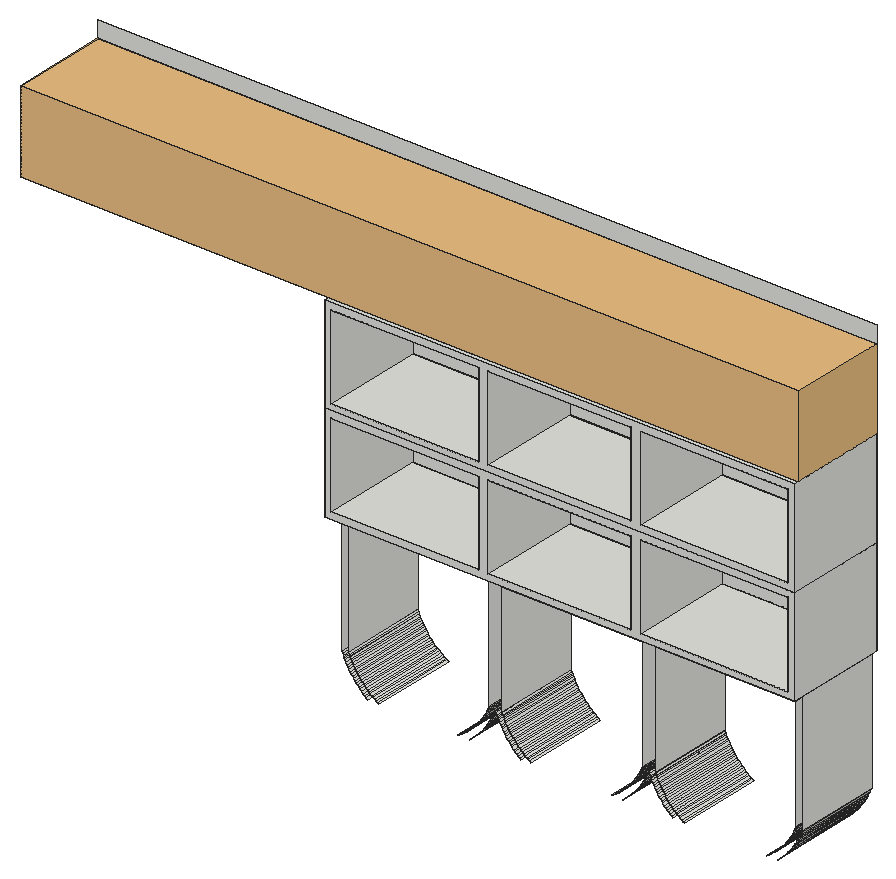
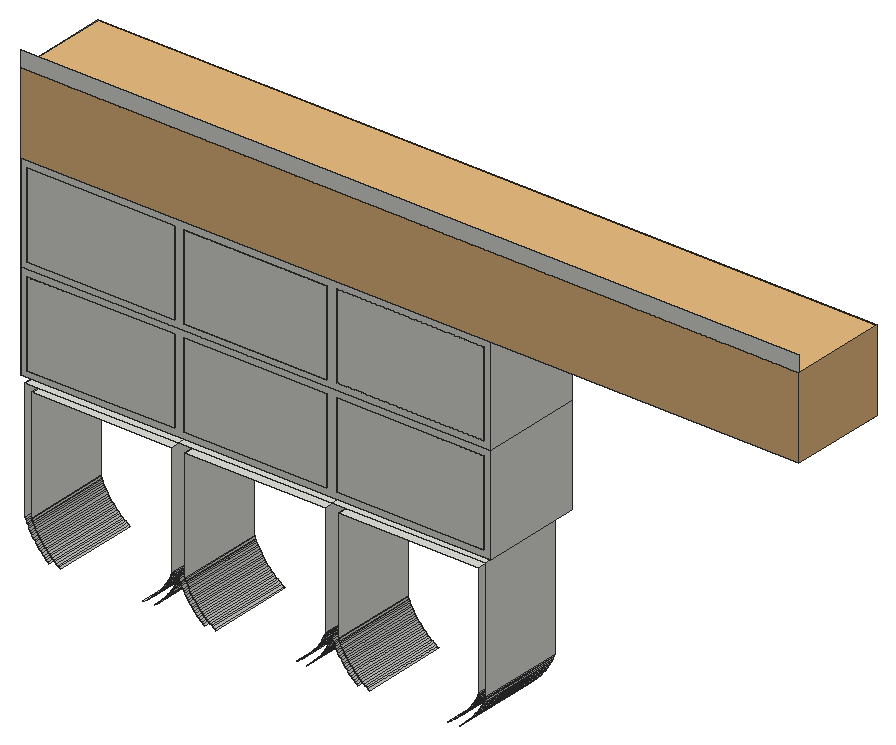
# SketchUp Ruby script. Lengths in inches.
U = 1.inch
M = Sketchup.active_model
def pt(a) = Geom::Point3d.new(a.map { |v| v * U })
def face(e, loops, mat)
  f = e.add_face(loops[0].map { |a| pt(a) })
  loops[1..].each { |l| e.add_face(l.map { |a| pt(a) }).erase! }
  f.material = f.back_material = mat if mat
  f
end
# faces: each face lists its corners as indices into pts; further lists are holes
def faces(e, pts, list, mat = nil) = list.each { |f| face(e, (f[0].is_a?(Array) ? f : [f]).map { |l| l.map { |i| pts[i] } }, mat) }
# xy, xz, yz: faces in a plane at the given z, y or x. An outline is a flat list of corners, or four numbers for a rectangle; further outlines are holes
def ring(l) = l.size == 4 ? [[l[0], l[1]], [l[2], l[1]], [l[2], l[3]], [l[0], l[3]]] : l.each_slice(2).to_a
def flat(e, list, mat, &to3) = list.each { |f| face(e, (f[0].is_a?(Array) ? f : [f]).map { |l| ring(l).map { |u, v| to3.(u, v) } }, mat) }
def xy(e, z, list, mat = nil) = flat(e, list, mat) { |x, y| [x, y, z] }
def xz(e, y, list, mat = nil) = flat(e, list, mat) { |x, z| [x, y, z] }
def yz(e, x, list, mat = nil) = flat(e, list, mat) { |y, z| [x, y, z] }
def lines(e, pts, list) = list.each { |a, b| e.add_line(pt(pts[a]), pt(pts[b])) }
# prism: a flat outline (further loops are holes) pulled along v
def prism(e, loops, v, mat = nil)
  f = face(e, loops, mat); d = Geom::Vector3d.new(v.map { |x| x * U })
  f.pushpull(f.normal.samedirection?(d) ? d.length : -d.length)
end
def box(e, o, s, mat = nil) = prism(e, [[o, [o[0] + s[0], o[1], o[2]], [o[0] + s[0], o[1] + s[1], o[2]], [o[0], o[1] + s[1], o[2]]]], [0, 0, s[2]], mat)
def at(x, y, z, deg = 0) = Geom::Transformation.translation(pt([x, y, z])) * Geom::Transformation.rotation(ORIGIN, Z_AXIS, deg.degrees)
def axes(o, x, y, z) = Geom::Transformation.new([*x, 0, *y, 0, *z, 0, *pt(o).to_a, 1])
def part(name) = M.definitions.add(name)
# library, detail: a bought-in or finely detailed component or shape, given as its bounding box
def library(name, o, s) = part(name).tap { |d| box(d.entities, o, s) }
def detail(e, o, s) = box(e.add_group.entities, o, s)
def put(e, d, t, mat = nil) = e.add_instance(d, t).tap { |i| i.material = mat if mat }
def group(e, t, mat = nil) = e.add_group.tap { |g| g.transformation = t; g.material = mat if mat }.entities
root = M.entities
c1 = library("Group\#5",[0,-12,0],[96,12,10])
xy(root,82.6,[[45.4,19.34,62.73,30],[64.33,19.34,81.67,30],[83.27,19.34,100.6,30]])
xy(root,83.4,[[44.6,19.34,63.53,30],[63.53,19.34,82.47,30],[82.47,19.34,101.4,30]])
xz(root,30,[[44.8,84.8,63,95.2],[64.2,84.8,81.8,95.2],[83,84.8,101.2,95.2],[6,118,102,120]])
yz(root,44.6,[[19.34,68.6,30,83.4]])
yz(root,45.4,[[19.34,68.75,30,82.6]])
yz(root,62.73,[[19.34,68.75,30,82.6]])
yz(root,64.33,[[19.34,68.75,30,82.6]])
yz(root,81.67,[[19.34,68.75,30,82.6]])
yz(root,83.27,[[19.34,68.75,30,82.6]])
yz(root,100.6,[[19.34,68.75,30,82.6]])
yz(root,101.4,[[19.34,68.6,30,83.4]])
p = [[47.59,30,64.45],[47.78,30,64.29],[47.78,19.34,64.29],[47.59,19.34,64.45],[49.21,30,64.28],[49.02,30,64.4],
  [49.02,19.34,64.4],[49.21,19.34,64.28],[59.11,30,64.4],[58.92,30,64.28],[58.92,19.34,64.28],[59.11,19.34,64.4],
  [60.35,30,64.29],[60.54,30,64.45],[60.54,19.34,64.45],[60.35,19.34,64.29],[66.52,30,64.4375],[66.71,30,64.28],
  [66.71,19.34,64.28],[66.52,19.34,64.4375],[78.05,30,64.38],[77.86,30,64.26],[77.86,19.34,64.26],[78.05,19.34,64.38],
  [79.29,30,64.28],[79.48,30,64.4375],[79.48,19.34,64.4375],[79.29,19.34,64.28],[86.87,30,64.34],[86.68,30,64.46],
  [86.68,19.34,64.46],[86.87,19.34,64.34],[97.19,30,64.46],[97,30,64.34],[97,19.34,64.34],[97.19,19.34,64.46],
  [47.4,30,64.61],[47.4,19.34,64.61],[48.83,30,64.52],[48.83,19.34,64.52],[59.3,30,64.52],[59.3,19.34,64.52],
  [60.73,30,64.61],[60.73,19.34,64.61],[66.33,30,64.6],[66.33,19.34,64.6],[67.95,30,64.38],[67.76,30,64.51],
  [67.76,19.34,64.51],[67.95,19.34,64.38],[78.24,30,64.51],[78.24,19.34,64.51],[79.67,30,64.6],[79.67,19.34,64.6],
  [85.25,30,64.5625],[85.4375,30,64.4],[85.4375,19.34,64.4],[85.25,19.34,64.5625],[98.43,30,64.4],[98.62,30,64.5625],
  [98.62,19.34,64.5625],[98.43,19.34,64.4],[48.64,30,64.65],[48.64,19.34,64.65],[59.49,30,64.65],[59.49,19.34,64.65],
  [67.57,30,64.64],[67.57,19.34,64.64],[78.43,30,64.64],[78.43,19.34,64.64],[86.49,30,64.59],[86.49,19.34,64.59],
  [97.375,30,64.59],[97.375,19.34,64.59],[47.22,30,64.77],[47.22,19.34,64.77],[60.91,30,64.77],[60.91,19.34,64.77],
  [66.15,30,64.76],[66.15,19.34,64.76],[67.39,30,64.77],[67.39,19.34,64.77],[78.61,30,64.77],[78.61,19.34,64.77],
  [79.85,30,64.76],[79.85,19.34,64.76],[85.06,30,64.73],[85.06,19.34,64.73],[86.31,30,64.73],[86.31,19.34,64.73],
  [97.56,30,64.73],[97.56,19.34,64.73],[98.8,30,64.73],[98.8,19.34,64.73],[48.46,30,64.78],[48.46,19.34,64.78],
  [59.67,30,64.78],[59.67,19.34,64.78],[84.89,30,64.9],[84.89,19.34,64.9],[86.125,30,64.87],[86.125,19.34,64.87],
  [97.74,30,64.87],[97.74,19.34,64.87],[98.98,30,64.9],[98.98,19.34,64.9],[47.04,30,64.94],[47.04,19.34,64.94],
  [48.28,30,64.92],[48.28,19.34,64.92],[59.85,30,64.92],[59.85,19.34,64.92],[61.09,30,64.94],[61.09,19.34,64.94],
  [65.97,30,64.93],[65.97,19.34,64.93],[67.21,30,64.91],[67.21,19.34,64.91],[78.79,30,64.91],[78.79,19.34,64.91],
  [80.03,30,64.93],[80.03,19.34,64.93],[46.87,30,65.11],[46.87,19.34,65.11],[48.1,30,65.07],[48.1,19.34,65.07],
  [60.03,30,65.07],[60.03,19.34,65.07],[61.27,30,65.11],[61.27,19.34,65.11],[65.79,30,65.1],[65.79,19.34,65.1],
  [67.03,30,65.05],[67.03,19.34,65.05],[78.97,30,65.05],[78.97,19.34,65.05],[80.21,30,65.1],[80.21,19.34,65.1],
  [84.71,30,65.07],[84.71,19.34,65.07],[85.95,30,65.01],[85.95,19.34,65.01],[97.92,30,65.01],[97.92,19.34,65.01],
  [99.16,30,65.07],[99.16,19.34,65.07],[85.78,30,65.16],[85.78,19.34,65.16],[98.09,30,65.16],[98.09,19.34,65.16],
  [46.69,30,65.29],[46.69,19.34,65.29],[47.93,30,65.21],[47.93,19.34,65.21],[60.2,30,65.21],[60.2,19.34,65.21],
  [61.44,30,65.29],[61.44,19.34,65.29],[65.62,30,65.28],[65.62,19.34,65.28],[66.86,30,65.2],[66.86,19.34,65.2],
  [79.14,30,65.2],[79.14,19.34,65.2],[80.38,30,65.28],[80.38,19.34,65.28],[84.54,30,65.25],[84.54,19.34,65.25],
  [99.33,30,65.25],[99.33,19.34,65.25],[47.76,30,65.36],[47.76,19.34,65.36],[60.375,30,65.36],[60.375,19.34,65.36],
  [66.6875,30,65.35],[66.6875,19.34,65.35],[79.3125,30,65.35],[79.3125,19.34,65.35],[85.61,30,65.32],[85.61,19.34,65.32],
  [98.26,30,65.32],[98.26,19.34,65.32],[46.53,30,65.47],[46.53,19.34,65.47],[61.61,30,65.47],[61.61,19.34,65.47],
  [65.45,30,65.46],[65.45,19.34,65.46],[80.55,30,65.46],[80.55,19.34,65.46],[84.37,30,65.4375],[84.37,19.34,65.4375],
  [85.44,30,65.47],[85.44,19.34,65.47],[98.42,30,65.47],[98.42,19.34,65.47],[99.49,30,65.4375],[99.49,19.34,65.4375],
  [47.59,30,65.52],[47.59,19.34,65.52],[60.54,30,65.52],[60.54,19.34,65.52],[66.52,30,65.51],[66.52,19.34,65.51],
  [79.48,30,65.51],[79.48,19.34,65.51],[84.21,30,65.625],[84.21,19.34,65.625],[99.66,30,65.625],[99.66,19.34,65.625],
  [46.36,30,65.66],[46.36,19.34,65.66],[47.43,30,65.68],[47.43,19.34,65.68],[60.7,30,65.68],[60.7,19.34,65.68],
  [61.77,30,65.66],[61.77,19.34,65.66],[65.29,30,65.65],[65.29,19.34,65.65],[66.36,30,65.67],[66.36,19.34,65.67],
  [79.64,30,65.67],[79.64,19.34,65.67],[80.71,30,65.65],[80.71,19.34,65.65],[85.28,30,65.63],[85.28,19.34,65.63],
  [98.59,30,65.63],[98.59,19.34,65.63],[65.13,30,65.84],[65.13,19.34,65.84],[80.87,30,65.84],[80.87,19.34,65.84],
  [84.05,30,65.81],[84.05,19.34,65.81],[85.125,30,65.8],[85.125,19.34,65.8],[98.74,30,65.8],[98.74,19.34,65.8],
  [99.8125,30,65.81],[99.8125,19.34,65.81],[46.21,30,65.84],[46.21,19.34,65.84],[47.27,30,65.84],[47.27,19.34,65.84],
  [60.86,30,65.84],[60.86,19.34,65.84],[61.93,30,65.84],[61.93,19.34,65.84],[66.2,30,65.83],[66.2,19.34,65.83],
  [79.8,30,65.83],[79.8,19.34,65.83],[46.05,30,66.04],[46.05,19.34,66.04],[47.12,30,66.01],[47.12,19.34,66.01],
  [61.01,30,66.01],[61.01,19.34,66.01],[62.08,30,66.04],[62.08,19.34,66.04],[64.98,30,66.03],[64.98,19.34,66.03],
  [66.05,30,66],[66.05,19.34,66],[79.95,30,66],[79.95,19.34,66],[81.02,30,66.03],[81.02,19.34,66.03],
  [83.9,30,66.01],[83.9,19.34,66.01],[84.97,30,65.97],[84.97,19.34,65.97],[98.9,30,65.97],[98.9,19.34,65.97],
  [99.97,30,66.01],[99.97,19.34,66.01],[45.9,30,66.23],[45.9,19.34,66.23],[46.97,30,66.18],[46.97,19.34,66.18],
  [61.16,30,66.18],[61.16,19.34,66.18],[62.23,30,66.23],[62.23,19.34,66.23],[64.83,30,66.23],[64.83,19.34,66.23],
  [65.9,30,66.17],[65.9,19.34,66.17],[80.1,30,66.17],[80.1,19.34,66.17],[81.17,30,66.23],[81.17,19.34,66.23],
  [83.75,30,66.21],[83.75,19.34,66.21],[84.82,30,66.14],[84.82,19.34,66.14],[99.05,30,66.14],[99.05,19.34,66.14],
  [100.11,30,66.21],[100.11,19.34,66.21],[84.68,30,66.32],[84.68,19.34,66.32],[99.19,30,66.32],[99.19,19.34,66.32],
  [45.76,30,66.43],[45.76,19.34,66.43],[46.83,30,66.35],[46.83,19.34,66.35],[61.31,30,66.35],[61.31,19.34,66.35],
  [62.375,30,66.43],[62.375,19.34,66.43],[64.6875,30,66.43],[64.6875,19.34,66.43],[65.75,30,66.34],[65.75,19.34,66.34],
  [80.25,30,66.34],[80.25,19.34,66.34],[81.3125,30,66.43],[81.3125,19.34,66.43],[83.61,30,66.41],[83.61,19.34,66.41],
  [100.26,30,66.41],[100.26,19.34,66.41],[65.61,30,66.52],[65.61,19.34,66.52],[80.39,30,66.52],[80.39,19.34,66.52],
  [84.54,30,66.5],[84.54,19.34,66.5],[99.33,30,66.5],[99.33,19.34,66.5],[45.62,30,66.64],[45.62,19.34,66.64],
  [46.68,30,66.53],[46.68,19.34,66.53],[61.45,30,66.53],[61.45,19.34,66.53],[62.51,30,66.64],[62.51,19.34,66.64],
  [64.55,30,66.63],[64.55,19.34,66.63],[81.45,30,66.63],[81.45,19.34,66.63],[83.47,30,66.62],[83.47,19.34,66.62],
  [100.4,30,66.62],[100.4,19.34,66.62],[46.55,30,66.71],[46.55,19.34,66.71],[61.59,30,66.71],[61.59,19.34,66.71],
  [65.48,30,66.7],[65.48,19.34,66.7],[80.52,30,66.7],[80.52,19.34,66.7],[84.4,30,66.68],[84.4,19.34,66.68],
  [99.47,30,66.68],[99.47,19.34,66.68],[45.49,30,66.84],[45.49,19.34,66.84],[62.65,30,66.84],[62.65,19.34,66.84],
  [64.42,30,66.84],[64.42,19.34,66.84],[81.58,30,66.84],[81.58,19.34,66.84],[83.34,30,66.82],[83.34,19.34,66.82],
  [100.53,30,66.82],[100.53,19.34,66.82],[46.41,30,66.89],[46.41,19.34,66.89],[61.72,30,66.89],[61.72,19.34,66.89],
  [65.34,30,66.89],[65.34,19.34,66.89],[80.66,30,66.89],[80.66,19.34,66.89],[84.27,30,66.86],[84.27,19.34,66.86],
  [99.6,30,66.86],[99.6,19.34,66.86],[45.36,30,67.05],[45.36,19.34,67.05],[62.78,30,67.05],[62.78,19.34,67.05],
  [64.29,30,67.05],[64.29,19.34,67.05],[81.71,30,67.05],[81.71,19.34,67.05],[83.21,30,67.04],[83.21,19.34,67.04],
  [100.66,30,67.04],[100.66,19.34,67.04],[46.29,30,67.08],[46.29,19.34,67.08],[61.85,30,67.08],[61.85,19.34,67.08],
  [65.22,30,67.07],[65.22,19.34,67.07],[80.78,30,67.07],[80.78,19.34,67.07],[84.14,30,67.05],[84.14,19.34,67.05],
  [99.73,30,67.05],[99.73,19.34,67.05],[64.16,30,67.26],[64.16,19.34,67.26],[81.84,30,67.26],[81.84,19.34,67.26],
  [83.09,30,67.25],[83.09,19.34,67.25],[100.78,30,67.25],[100.78,19.34,67.25],[45.23,30,67.27],[45.23,19.34,67.27],
  [46.16,30,67.27],[46.16,19.34,67.27],[61.97,30,67.27],[61.97,19.34,67.27],[62.9,30,67.27],[62.9,19.34,67.27],
  [65.09,30,67.27],[65.09,19.34,67.27],[80.91,30,67.27],[80.91,19.34,67.27],[84.02,30,67.25],[84.02,19.34,67.25],
  [99.85,30,67.25],[99.85,19.34,67.25],[83.9,30,67.44],[83.9,19.34,67.44],[99.97,30,67.44],[99.97,19.34,67.44],
  [45.11,30,67.48],[45.11,19.34,67.48],[46.04,30,67.46],[46.04,19.34,67.46],[62.09,30,67.46],[62.09,19.34,67.46],
  [63.02,30,67.48],[63.02,19.34,67.48],[64.04,30,67.48],[64.04,19.34,67.48],[64.97,30,67.46],[64.97,19.34,67.46],
  [81.03,30,67.46],[81.03,19.34,67.46],[81.96,30,67.48],[81.96,19.34,67.48],[82.97,30,67.47],[82.97,19.34,67.47],
  [100.9,30,67.47],[100.9,19.34,67.47],[83.79,30,67.64],[83.79,19.34,67.64],[100.08,30,67.64],[100.08,19.34,67.64],
  [45,30,67.7],[45,19.34,67.7],[45.93,30,67.66],[45.93,19.34,67.66],[62.2,30,67.66],[62.2,19.34,67.66],
  [63.13,30,67.7],[63.13,19.34,67.7],[63.93,30,67.7],[63.93,19.34,67.7],[64.86,30,67.66],[64.86,19.34,67.66],
  [81.14,30,67.66],[81.14,19.34,67.66],[82.07,30,67.7],[82.07,19.34,67.7],[82.86,30,67.69],[82.86,19.34,67.69],
  [101.01,30,67.69],[101.01,19.34,67.69],[83.68,30,67.84],[83.68,19.34,67.84],[100.1875,30,67.84],[100.1875,19.34,67.84],
  [44.89,30,67.92],[44.89,19.34,67.92],[45.82,30,67.86],[45.82,19.34,67.86],[62.3125,30,67.86],[62.3125,19.34,67.86],
  [63.24,30,67.92],[63.24,19.34,67.92],[63.82,30,67.92],[63.82,19.34,67.92],[64.75,30,67.85],[64.75,19.34,67.85],
  [81.25,30,67.85],[81.25,19.34,67.85],[82.18,30,67.92],[82.18,19.34,67.92],[82.75,30,67.91],[82.75,19.34,67.91],
  [101.11,30,67.91],[101.11,19.34,67.91],[83.58,30,68.04],[83.58,19.34,68.04],[100.29,30,68.04],[100.29,19.34,68.04],
  [44.86,30,68],[44.86,19.34,68],[45.71,30,68.06],[45.71,19.34,68.06],[62.42,30,68.06],[62.42,19.34,68.06],
  [63.28,30,68],[63.28,19.34,68],[63.79,30,68],[63.79,19.34,68],[64.65,30,68.06],[64.65,19.34,68.06],
  [81.35,30,68.06],[81.35,19.34,68.06],[82.21,30,68],[82.21,19.34,68],[82.71,30,68],[82.71,19.34,68],
  [101.15,30,68],[101.15,19.34,68],[44.79,30,68.15],[44.79,19.34,68.15],[63.34,30,68.15],[63.34,19.34,68.15],
  [63.72,30,68.14],[63.72,19.34,68.14],[82.28,30,68.14],[82.28,19.34,68.14],[82.65,30,68.14],[82.65,19.34,68.14],
  [83.48,30,68.25],[83.48,19.34,68.25],[100.39,30,68.25],[100.39,19.34,68.25],[101.21,30,68.14],[101.21,19.34,68.14],
  [44.69,30,68.37],[44.69,19.34,68.37],[45.61,30,68.26],[45.61,19.34,68.26],[62.52,30,68.26],[62.52,19.34,68.26],
  [63.44,30,68.37],[63.44,19.34,68.37],[63.625,30,68.37],[63.625,19.34,68.37],[64.55,30,68.26],[64.55,19.34,68.26],
  [81.45,30,68.26],[81.45,19.34,68.26],[82.375,30,68.37],[82.375,19.34,68.37],[82.56,30,68.37],[82.56,19.34,68.37],
  [101.31,30,68.37],[101.31,19.34,68.37],[83.45,30,68.33],[83.45,19.34,68.33],[100.42,30,68.33],[100.42,19.34,68.33],
  [45.58,30,68.33],[45.52,30,68.47],[45.52,19.34,68.47],[45.58,19.34,68.33],[62.55,30,68.33],[62.55,19.34,68.33],
  [62.61,30,68.47],[62.61,19.34,68.47],[64.52,30,68.33],[64.52,19.34,68.33],[64.45,30,68.47],[64.45,19.34,68.47],
  [81.48,30,68.33],[81.48,19.34,68.33],[81.55,30,68.47],[81.55,19.34,68.47],[83.39,30,68.46],[83.39,19.34,68.46],
  [100.48,30,68.46],[100.48,19.34,68.46],[44.6,30,68.6],[44.6,19.34,68.6],[63.53,30,68.6],[63.53,19.34,68.6],
  [82.47,30,68.6],[82.47,19.34,68.6],[101.4,30,68.6],[101.4,19.34,68.6],[45.43,30,68.68],[45.43,19.34,68.68],
  [62.7,30,68.68],[62.7,19.34,68.68],[64.36,30,68.68],[64.36,19.34,68.68],[81.64,30,68.68],[81.64,19.34,68.68],
  [83.3,30,68.67],[83.3,19.34,68.67],[100.57,30,68.67],[100.57,19.34,68.67],[45.4,30,68.75],[45.4,19.34,68.75],
  [62.73,30,68.75],[62.73,19.34,68.75],[64.33,30,68.75],[64.33,19.34,68.75],[81.67,30,68.75],[81.67,19.34,68.75],
  [83.27,30,68.75],[83.27,19.34,68.75],[100.6,30,68.75],[100.6,19.34,68.75]]
faces(root,p,[[0,1,2,3],[4,5,6,7],[8,9,10,11],[12,13,14,15],[16,17,18,19],[20,21,22,23],[24,25,26,27],[28,29,30,31],
  [32,33,34,35],[36,0,3,37],[5,38,39,6],[40,8,11,41],[13,42,43,14],[44,16,19,45],[46,47,48,49],[50,20,23,51],
  [25,52,53,26],[54,55,56,57],[58,59,60,61],[38,62,63,39],[64,40,41,65],[47,66,67,48],[68,50,51,69],[29,70,71,30],
  [72,32,35,73],[74,36,37,75],[42,76,77,43],[78,44,45,79],[66,80,81,67],[82,68,69,83],[52,84,85,53],[86,54,57,87],
  [70,88,89,71],[90,72,73,91],[59,92,93,60],[62,94,95,63],[96,64,65,97],[98,86,87,99],[88,100,101,89],[102,90,91,103],
  [92,104,105,93],[106,74,75,107],[94,108,109,95],[110,96,97,111],[76,112,113,77],[114,78,79,115],[80,116,117,81],[118,82,83,119],
  [84,120,121,85],[122,106,107,123],[108,124,125,109],[126,110,111,127],[112,128,129,113],[130,114,115,131],[116,132,133,117],[134,118,119,135],
  [120,136,137,121],[138,98,99,139],[100,140,141,101],[142,102,103,143],[104,144,145,105],[140,146,147,141],[148,142,143,149],[150,122,123,151],
  [124,152,153,125],[154,126,127,155],[128,156,157,129],[158,130,131,159],[132,160,161,133],[162,134,135,163],[136,164,165,137],[166,138,139,167],
  [144,168,169,145],[152,170,171,153],[172,154,155,173],[160,174,175,161],[176,162,163,177],[146,178,179,147],[180,148,149,181],[182,150,151,183],
  [156,184,185,157],[186,158,159,187],[164,188,189,165],[190,166,167,191],[178,192,193,179],[194,180,181,195],[168,196,197,169],[170,198,199,171],
  [200,172,173,201],[174,202,203,175],[204,176,177,205],[206,190,191,207],[196,208,209,197],[210,182,183,211],[198,212,213,199],[214,200,201,215],
  [184,216,217,185],[218,186,187,219],[202,220,221,203],[222,204,205,223],[188,224,225,189],[192,226,227,193],[228,194,195,229],[230,218,219,231],
  [224,232,233,225],[234,206,207,235],[226,236,237,227],[238,228,229,239],[208,240,241,209],[242,210,211,243],[212,244,245,213],[246,214,215,247],
  [216,248,249,217],[220,250,251,221],[252,222,223,253],[254,242,243,255],[244,256,257,245],[258,246,247,259],[248,260,261,249],[262,230,231,263],
  [250,264,265,251],[266,252,253,267],[232,268,269,233],[270,234,235,271],[236,272,273,237],[274,238,239,275],[240,276,277,241],[278,254,255,279],
  [256,280,281,257],[282,258,259,283],[260,284,285,261],[286,262,263,287],[264,288,289,265],[290,266,267,291],[268,292,293,269],[294,270,271,295],
  [272,296,297,273],[298,274,275,299],[276,300,301,277],[296,302,303,297],[304,298,299,305],[306,278,279,307],[280,308,309,281],[310,282,283,311],
  [284,312,313,285],[314,286,287,315],[288,316,317,289],[318,290,291,319],[292,320,321,293],[322,294,295,323],[300,324,325,301],[316,326,327,317],
  [328,318,319,329],[302,330,331,303],[332,304,305,333],[334,306,307,335],[308,336,337,309],[338,310,311,339],[312,340,341,313],[342,314,315,343],
  [320,344,345,321],[346,322,323,347],[324,348,349,325],[336,350,351,337],[352,338,339,353],[326,354,355,327],[356,328,329,357],[330,358,359,331],
  [360,332,333,361],[362,334,335,363],[340,364,365,341],[366,342,343,367],[344,368,369,345],[370,346,347,371],[348,372,373,349],[350,374,375,351],
  [376,352,353,377],[354,378,379,355],[380,356,357,381],[358,382,383,359],[384,360,361,385],[386,362,363,387],[364,388,389,365],[390,366,367,391],
  [368,392,393,369],[394,370,371,395],[372,396,397,373],[374,398,399,375],[400,376,377,401],[378,402,403,379],[404,380,381,405],[382,406,407,383],
  [408,384,385,409],[410,390,391,411],[392,412,413,393],[414,394,395,415],[396,416,417,397],[418,386,387,419],[398,420,421,399],[422,400,401,423],
  [388,424,425,389],[402,426,427,403],[428,404,405,429],[406,430,431,407],[432,408,409,433],[430,434,435,431],[436,432,433,437],[438,418,419,439],
  [420,440,441,421],[442,422,423,443],[424,444,445,425],[446,410,411,447],[426,448,449,427],[450,428,429,451],[412,452,453,413],[454,414,415,455],
  [416,456,457,417],[434,458,459,435],[460,436,437,461],[462,438,439,463],[440,464,465,441],[466,442,443,467],[444,468,469,445],[470,446,447,471],
  [448,472,473,449],[474,450,451,475],[452,476,477,453],[478,454,455,479],[456,480,481,457],[458,482,483,459],[484,460,461,485],[486,462,463,487],
  [464,488,489,465],[490,466,467,491],[468,492,493,469],[494,470,471,495],[472,496,497,473],[498,474,475,499],[476,500,501,477],[502,478,479,503],
  [480,504,505,481],[482,506,507,483],[508,484,485,509],[510,486,487,511],[488,512,513,489],[514,490,491,515],[492,516,517,493],[518,494,495,519],
  [496,520,521,497],[522,498,499,523],[500,524,525,501],[526,502,503,527],[504,528,529,505],[530,510,511,531],[516,532,533,517],[534,518,519,535],
  [524,536,537,525],[538,526,527,539],[506,540,541,507],[542,508,509,543],[528,544,545,529],[546,530,531,547],[512,548,549,513],[550,514,515,551],
  [532,552,553,533],[554,534,535,555],[520,556,557,521],[558,522,523,559],[536,560,561,537],[562,538,539,563],[544,564,565,545],[540,566,567,541],
  [568,542,543,569],[570,571,572,573],[548,570,573,549],[574,550,551,575],[576,574,575,577],[556,578,579,557],[578,580,581,579],[582,558,559,583],
  [584,582,583,585],[566,586,587,567],[588,568,569,589],[590,546,547,591],[552,592,593,553],[592,554,555,593],[560,594,595,561],[594,562,563,595],
  [564,596,597,565],[571,598,599,572],[600,576,577,601],[580,602,603,581],[604,584,585,605],[586,606,607,587],[608,588,589,609],[598,610,611,599],
  [612,600,601,613],[602,614,615,603],[616,604,605,617],[606,618,619,607],[620,608,609,621]])
g1 = group(root,at(44,30,84))
prism(g1,[[[0,0,0],[0,0,12],[58,0,12],[58,0,0]],[[39,0,0.8],[57.2,0,0.8],[57.2,0,11.2],[39,0,11.2]],[[19,0,0.8],[19,0,11.2],[0.8,0,11.2],[0.8,0,0.8]],[[37.8,0,0.8],[37.8,0,11.2],[20.2,0,11.2],[20.2,0,0.8]]],[0,-12.6,0])
g2 = group(root,at(44,30,96))
xy(g2,0,[[0,-12.6,58,0]])
xy(g2,0.8,[[0.8,-12.6,19,0],[20.2,-12.6,37.8,0],[39,-12.6,57.2,0]])
xy(g2,11.2,[[0.8,-12.6,19,0],[20.2,-12.6,37.8,0],[39,-12.6,57.2,0]])
xy(g2,12,[[0,-12.6,58,0]])
xz(g2,-12.6,[[[0,0,58,12],[39,0.8,57.2,11.2],[0.8,0.8,19,11.2],[20.2,0.8,37.8,11.2]]])
xz(g2,0,[[[0,0,58,12],[39,0.8,57.2,11.2],[0.8,0.8,19,11.2],[20.2,0.8,37.8,11.2]],[0.8,0.8,19,11.2],[20.2,0.8,37.8,11.2],[39,0.8,57.2,11.2]])
yz(g2,0,[[-12.6,0,0,12]])
yz(g2,0.8,[[-12.6,0.8,0,11.2]])
yz(g2,19,[[-12.6,0.8,0,11.2]])
yz(g2,20.2,[[-12.6,0.8,0,11.2]])
yz(g2,37.8,[[-12.6,0.8,0,11.2]])
yz(g2,39,[[-12.6,0.8,0,11.2]])
yz(g2,57.2,[[-12.6,0.8,0,11.2]])
yz(g2,58,[[-12.6,0,0,12]])
put(root,c1,at(6,30,108))
